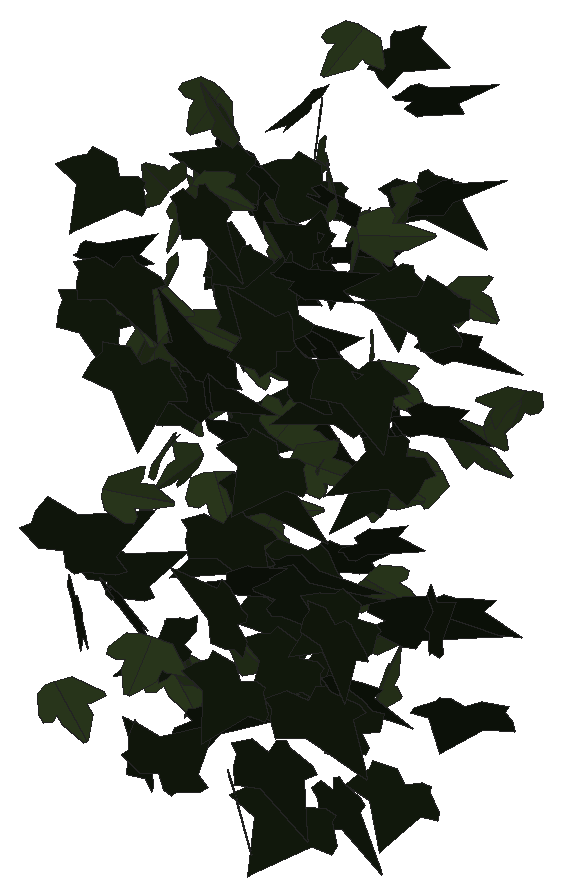
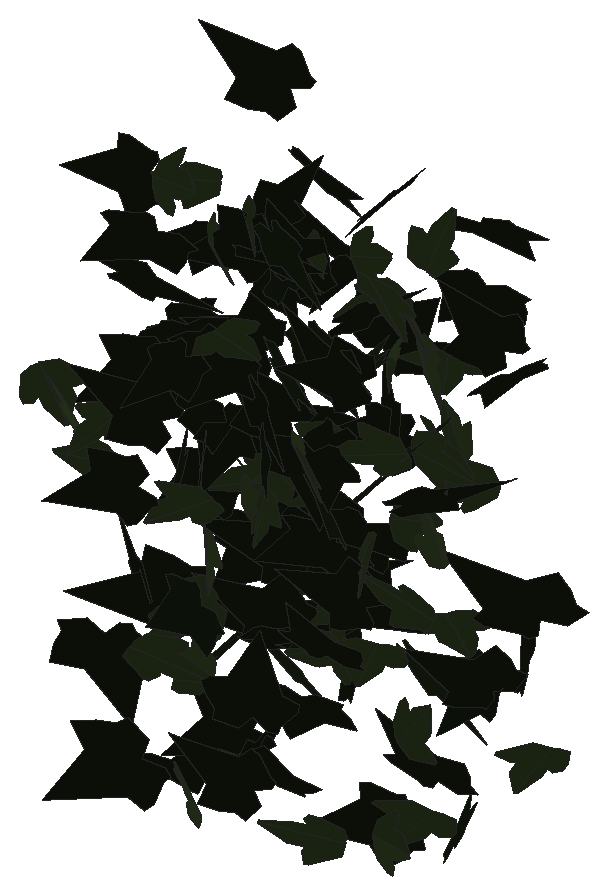
# SketchUp Ruby script. Lengths in inches.
U = 1.inch
M = Sketchup.active_model
def pt(a) = Geom::Point3d.new(a.map { |v| v * U })
def face(e, loops, mat)
  f = e.add_face(loops[0].map { |a| pt(a) })
  loops[1..].each { |l| e.add_face(l.map { |a| pt(a) }).erase! }
  f.material = f.back_material = mat if mat
  f
end
# faces: each face lists its corners as indices into pts; further lists are holes
def faces(e, pts, list, mat = nil) = list.each { |f| face(e, (f[0].is_a?(Array) ? f : [f]).map { |l| l.map { |i| pts[i] } }, mat) }
# xy, xz, yz: faces in a plane at the given z, y or x. An outline is a flat list of corners, or four numbers for a rectangle; further outlines are holes
def ring(l) = l.size == 4 ? [[l[0], l[1]], [l[2], l[1]], [l[2], l[3]], [l[0], l[3]]] : l.each_slice(2).to_a
def flat(e, list, mat, &to3) = list.each { |f| face(e, (f[0].is_a?(Array) ? f : [f]).map { |l| ring(l).map { |u, v| to3.(u, v) } }, mat) }
def xy(e, z, list, mat = nil) = flat(e, list, mat) { |x, y| [x, y, z] }
def xz(e, y, list, mat = nil) = flat(e, list, mat) { |x, z| [x, y, z] }
def yz(e, x, list, mat = nil) = flat(e, list, mat) { |y, z| [x, y, z] }
def lines(e, pts, list) = list.each { |a, b| e.add_line(pt(pts[a]), pt(pts[b])) }
# prism: a flat outline (further loops are holes) pulled along v
def prism(e, loops, v, mat = nil)
  f = face(e, loops, mat); d = Geom::Vector3d.new(v.map { |x| x * U })
  f.pushpull(f.normal.samedirection?(d) ? d.length : -d.length)
end
def box(e, o, s, mat = nil) = prism(e, [[o, [o[0] + s[0], o[1], o[2]], [o[0] + s[0], o[1] + s[1], o[2]], [o[0], o[1] + s[1], o[2]]]], [0, 0, s[2]], mat)
def at(x, y, z, deg = 0) = Geom::Transformation.translation(pt([x, y, z])) * Geom::Transformation.rotation(ORIGIN, Z_AXIS, deg.degrees)
def axes(o, x, y, z) = Geom::Transformation.new([*x, 0, *y, 0, *z, 0, *pt(o).to_a, 1])
def part(name) = M.definitions.add(name)
# library, detail: a bought-in or finely detailed component or shape, given as its bounding box
def library(name, o, s) = part(name).tap { |d| box(d.entities, o, s) }
def detail(e, o, s) = box(e.add_group.entities, o, s)
def put(e, d, t, mat = nil) = e.add_instance(d, t).tap { |i| i.material = mat if mat }
def group(e, t, mat = nil) = e.add_group.tap { |g| g.transformation = t; g.material = mat if mat }.entities
root = M.entities
M.materials.add("1026 AP 7946 SUNNY SIDE UP").color = [254, 231, 186]
M.materials.add("efeu1").color = [18, 25, 13]
M.materials.add("efeu2").color = [43, 57, 29]
c1 = part("ivyleaf_10")
p = [[0,0.5,-0.03],[-0.0625,2.02,-0.43],[-0.19,2.01,-0.46],[-0.54,1.05,-0.29],[-0.52,0.625,-0.18],[-0.83,0.76,-0.28],
  [-1.16,0.64,-0.33],[-1.15,0.33,-0.24],[-0.77,-0.39,0.02],[-0.3,-0.51,0.16],[0.04,-0.48,0.23],[-0.02,2.01,-0.4375],
  [-0.06,2.01,-0.43],[0.04,-0.49,0.23],[0.67,-0.49,0.14],[1.38,0.36,-0.2],[1.375,0.51,-0.24],[0.81,0.65,-0.19],
  [0.62,0.59,-0.15],[0.6,1.09,-0.28],[0.5,1.23,-0.31]]
faces(c1.entities,p,[[0,1,2,3,4,5,6,7,8,9,10],[11,12,0,13,14,15,16,17,18,19,20]],"efeu2")
c2 = part("ivyleaf_9")
p = [[1.54,2.16,1.25],[1.36,2.04,1.19],[-0.21,0.99,0.68],[-0.71,1.11,0.82],[-0.85,0.86,0.67],[-0.8,0.17,0.21],
  [-0.9,-0.01,0.1],[-0.67,-0.16,-0.02],[-0.08,-0.08,-0.05],[-0.03,-0.6,-0.4],[0.65,-0.88,-0.66],[0.83,-0.6,-0.49],
  [1.29,-0.42,-0.43],[1.8125,-0.07,-0.26],[1.21,0.44,0.15]]
faces(c2.entities,p,[[0,1,2,3,4,5,6,7,8,9,10,11,12,13,14]],"efeu1")
put(root,c1,axes([150.24,214.86,288],[0.00034,-0.24458,-0.28841],[0.01461,0.27848,-0.25025],[0.58271,-0.00684,0.00644]),"1026 AP 7946 SUNNY SIDE UP")
put(root,c1,axes([150.29,212.04,290.43],[0.54174,-0.1658,-0.09106],[-0.13351,0.0251,-0.39349],[0.26277,0.35457,-0.01218]),"1026 AP 7946 SUNNY SIDE UP")
put(root,c2,axes([149.95,209.48,288.4],[0.45459,0.23395,-0.02201],[-0.00198,0.03751,0.38211],[0.36958,-0.28756,0.02911]),"1026 AP 7946 SUNNY SIDE UP")
put(root,c2,axes([150.08,209.08,287.71],[0.00627,-0.39476,-0.09926],[0.00472,0.09414,-0.40613],[0.6381,0.00318,0.00398]),"1026 AP 7946 SUNNY SIDE UP")
put(root,c1,axes([150.71,210.34,286.64],[-0.04708,-0.01723,-0.40837],[-0.50973,0.23012,0.01627],[0.35949,0.32404,-0.03041]),"1026 AP 7946 SUNNY SIDE UP")
put(root,c1,axes([149.87,213.81,281.72],[0.10364,-0.0263,-0.38331],[0.56164,0.11278,0.05766],[0.16815,-0.36049,0.04368]),"1026 AP 7946 SUNNY SIDE UP")
put(root,c1,axes([150.11,208.24,280.67],[0.29267,0.32134,0.13775],[0.1212,0.10769,-0.38173],[-0.53256,0.2011,-0.01118]),"1026 AP 7946 SUNNY SIDE UP")
put(root,c1,axes([149.9,211.58,284.72],[0.1979,-0.0697,-0.35915],[0.53898,-0.07279,0.14221],[-0.14605,-0.36305,0.03816]),"1026 AP 7946 SUNNY SIDE UP")
put(root,c2,axes([150.51,209.19,290.25],[-0.54504,-0.1927,-0.01598],[0.05045,-0.0282,-0.40663],[0.29963,-0.34578,0.0394]),"1026 AP 7946 SUNNY SIDE UP")
put(root,c2,axes([149.99,208.55,283.28],[-0.17111,0.04006,0.48252],[0.73686,-0.02559,0.11433],[0.05358,0.47995,-0.03134]),"1026 AP 7946 SUNNY SIDE UP")
put(root,c1,axes([150.58,211.34,288.83],[-0.03018,0.18451,-0.32659],[-0.14274,0.30626,0.19046],[0.56028,0.08796,0.03093]),"1026 AP 7946 SUNNY SIDE UP")
put(root,c2,axes([150.23,214.96,288.8125],[-0.09888,-0.02115,-0.37658],[0.4884,-0.19924,-0.04435],[-0.3045,-0.31271,0.05115]),"1026 AP 7946 SUNNY SIDE UP")
put(root,c2,axes([150.18,209.46,282.35],[-0.04219,0.03422,0.41272],[0.61861,0.08419,0.02024],[-0.12905,0.3924,-0.03791]),"1026 AP 7946 SUNNY SIDE UP")
put(root,c2,axes([150.21,208.48,282.41],[0.17647,-0.13219,-0.39528],[0.52913,-0.19083,0.16834],[-0.35468,-0.35046,0.05448]),"1026 AP 7946 SUNNY SIDE UP")
put(root,c2,axes([150.96,210.46,285.75],[-0.2897,-0.40546,-0.16511],[-0.13991,-0.13281,0.45733],[-0.66977,0.20312,-0.02412]),"1026 AP 7946 SUNNY SIDE UP")
put(root,c1,axes([150.59,209.72,286.52],[0.02737,-0.37422,-0.00824],[0.00724,-0.00567,0.38588],[-0.58846,-0.01748,0.00436]),"1026 AP 7946 SUNNY SIDE UP")
put(root,c2,axes([150.47,209.22,282.26],[0.55635,-0.13712,-0.12245],[-0.19009,0.01383,-0.38967],[0.21172,0.37275,-0.02811]),"1026 AP 7946 SUNNY SIDE UP")
put(root,c2,axes([150.28,212.57,289.06],[0.42377,-0.12014,0.22844],[0.30943,-0.10439,-0.30434],[0.24953,0.33349,-0.01057]),"1026 AP 7946 SUNNY SIDE UP")
put(root,c1,axes([150.6,210.05,286.77],[0.51821,-0.16541,0.14391],[0.17496,-0.09084,-0.37922],[0.29316,0.34661,-0.02808]),"1026 AP 7946 SUNNY SIDE UP")
put(root,c1,axes([150.82,210.6,289.13],[0.3492,-0.30517,0.07536],[0.04115,-0.07341,-0.38861],[0.49237,0.22257,-0.02097]),"1026 AP 7946 SUNNY SIDE UP")
put(root,c1,axes([151.16,211.37,290.43],[-0.20983,0.13808,-0.3234],[-0.33943,0.22901,0.19915],[0.42048,0.25377,-0.00062]),"1026 AP 7946 SUNNY SIDE UP")
put(root,c2,axes([150.6,210.57,287],[0.10705,-0.39481,0.05601],[0.00608,-0.05678,-0.41303],[0.62712,0.06795,-0.00556]),"1026 AP 7946 SUNNY SIDE UP")
put(root,c1,axes([150.93,211.48,285.47],[-0.25567,0.31194,0.16328],[-0.1495,0.12678,-0.36084],[-0.52816,-0.18689,0.0231]),"1026 AP 7946 SUNNY SIDE UP")
put(root,c1,axes([150.9375,209.99,289.87],[-0.14488,-0.27499,-0.27658],[-0.16628,-0.24561,0.29686],[-0.57918,0.1393,-0.01604]),"1026 AP 7946 SUNNY SIDE UP")
put(root,c1,axes([150.96,210.08,288.21],[0.17104,-0.3806,-0.06422],[-0.05174,0.05313,-0.40711],[0.60368,0.11239,-0.01669]),"1026 AP 7946 SUNNY SIDE UP")
put(root,c2,axes([151.11,212.31,286.45],[0.00976,0.18092,0.35437],[-0.05752,0.34175,-0.18304],[-0.60699,-0.02948,0.02305]),"1026 AP 7946 SUNNY SIDE UP")
put(root,c1,axes([150.63,210.48,280.4],[0.45779,0.21342,0.1689],[0.24019,0.06566,-0.36984],[-0.347,0.32701,-0.03317]),"1026 AP 7946 SUNNY SIDE UP")
put(root,c2,axes([151.17,211.74,289.44],[-0.06207,-0.33555,-0.20129],[0.00563,-0.19479,0.34613],[-0.60902,0.0324,0.02372]),"1026 AP 7946 SUNNY SIDE UP")
put(root,c1,axes([151.09,214.87,290.61],[0.32558,0.21594,-0.25711],[-0.23061,-0.20533,-0.30807],[-0.4665,0.25221,-0.02714]),"1026 AP 7946 SUNNY SIDE UP")
put(root,c1,axes([150.86,209.91,284.68],[0.09622,-0.35154,-0.13633],[0.10498,-0.11973,0.36429],[-0.58011,-0.07998,0.04331]),"1026 AP 7946 SUNNY SIDE UP")
put(root,c1,axes([150.99,211.06,280.11],[0.1059,-0.23251,0.30563],[0.11783,-0.28846,-0.251],[0.58252,0.10062,-0.00479]),"1026 AP 7946 SUNNY SIDE UP")
put(root,c2,axes([150.93,209.38,279.36],[-0.0516,-0.14945,0.37337],[-0.07555,-0.36028,-0.15927],[0.61303,-0.05698,0.0118]),"1026 AP 7946 SUNNY SIDE UP")
put(root,c1,axes([150.91,209.57,287.91],[0.48108,0.21701,0.02587],[0.05927,-0.01202,-0.38513],[-0.33813,0.30665,-0.03071]),"1026 AP 7946 SUNNY SIDE UP")
put(root,c2,axes([150.96,212.49,284.02],[-0.41082,0.1446,0.22534],[0.32976,-0.06821,0.30525],[0.2457,0.33331,-0.03289]),"1026 AP 7946 SUNNY SIDE UP")
put(root,c2,axes([151.13,215.4,286.07],[-0.18298,0.24576,-0.30283],[-0.16397,0.27681,0.28124],[0.58148,0.15539,-0.01599]),"1026 AP 7946 SUNNY SIDE UP")
put(root,c1,axes([150.94,211.35,283.58],[0.45385,0.25447,0.08235],[0.12239,0.03009,-0.39516],[-0.40045,0.2976,-0.02744]),"1026 AP 7946 SUNNY SIDE UP")
put(root,c2,axes([150.875,208.71,288.81],[-0.22082,-0.19079,-0.33081],[0.34068,0.23642,-0.24176],[0.47662,-0.25738,0.01955]),"1026 AP 7946 SUNNY SIDE UP")
put(root,c2,axes([150.77,212.36,288.68],[-0.05022,0.0705,0.4441],[0.37785,-0.35763,0.07658],[0.57282,0.24209,-0.01158]),"1026 AP 7946 SUNNY SIDE UP")
put(root,c1,axes([151.26,212.72,287.52],[0.36743,-0.32066,0.03108],[0.00066,-0.03922,-0.40831],[0.5067,0.23257,-0.02201]),"1026 AP 7946 SUNNY SIDE UP")
put(root,c1,axes([151.07,210.81,289.52],[-0.19708,-0.15266,-0.31964],[0.3999,0.18157,-0.19736],[0.3666,-0.28013,0.04345]),"1026 AP 7946 SUNNY SIDE UP")
put(root,c2,axes([151.29,211.375,288.16],[-0.2015,-0.26233,0.30728],[-0.06883,-0.30371,-0.29487],[0.62256,-0.11848,0.06685]),"1026 AP 7946 SUNNY SIDE UP")
put(root,c2,axes([151.48,212.14,287.16],[0.30508,0.27098,-0.16444],[-0.14239,-0.13335,-0.3441],[-0.47485,0.21408,-0.00246]),"1026 AP 7946 SUNNY SIDE UP")
put(root,c1,axes([151.01,210.85,286.8],[0.13389,0.09764,0.36147],[0.43736,0.2143,-0.12993],[-0.3684,0.28991,-0.02289]),"1026 AP 7946 SUNNY SIDE UP")
put(root,c1,axes([151.7,209.58,281.05],[-0.44068,0.20269,-0.19714],[-0.21039,0.14208,0.35561],[0.38593,0.3089,-0.03125]),"1026 AP 7946 SUNNY SIDE UP")
put(root,c2,axes([151.46,211.36,288.15],[-0.25654,-0.18391,0.34807],[-0.09845,-0.35048,-0.22904],[0.59826,-0.13654,0.11156]),"1026 AP 7946 SUNNY SIDE UP")
put(root,c2,axes([151.44,215.4,290.29],[0.03416,-0.00028,-0.40229],[-0.16016,0.37756,-0.0039],[0.59276,0.10203,0.02213]),"1026 AP 7946 SUNNY SIDE UP")
put(root,c2,axes([151.05,211.49,284.39],[0.29873,-0.08382,0.32586],[0.43791,-0.15166,-0.21429],[0.27152,0.33682,-0.0129]),"1026 AP 7946 SUNNY SIDE UP")
put(root,c1,axes([151.59,209.82,284.95],[0.01963,-0.11739,0.37353],[0.04799,-0.36198,-0.1237],[0.59834,0.03288,-0.00233]),"1026 AP 7946 SUNNY SIDE UP")
put(root,c1,axes([151.35,208.21,284.95],[0.05812,0.09763,0.39619],[0.18914,0.36472,-0.10532],[-0.59365,0.12576,0.00523]),"1026 AP 7946 SUNNY SIDE UP")
put(root,c2,axes([151.54,213.5625,283.24],[0.5902,-0.11463,0.14851],[-0.18939,0.09673,0.40106],[-0.22015,-0.39052,0.05313]),"1026 AP 7946 SUNNY SIDE UP")
put(root,c2,axes([152.08,208.95,281.98],[-0.52423,0.31035,-0.04182],[0.01308,-0.05307,-0.46832],[-0.49235,-0.33186,0.03209]),"1026 AP 7946 SUNNY SIDE UP")
put(root,c2,axes([151.52,210.0625,279.86],[0.06074,0.21571,-0.37049],[0.04708,0.36004,0.22714],[0.65938,-0.04558,0.01791]),"1026 AP 7946 SUNNY SIDE UP")
put(root,c2,axes([151.68,208.4,287.38],[-0.27135,-0.41978,-0.06538],[0.05889,0.05061,-0.46701],[0.66442,-0.17592,0.01469]),"1026 AP 7946 SUNNY SIDE UP")
put(root,c2,axes([151.88,211.18,286.92],[0.0224,-0.07632,-0.39385],[-0.27179,0.34119,-0.0749],[0.54872,0.17211,-0.02102]),"1026 AP 7946 SUNNY SIDE UP")
put(root,c2,axes([152.14,212.28,290.83],[-0.28555,0.31398,-0.0678],[0.03102,-0.0666,-0.37369],[-0.50406,-0.18197,0.01541]),"1026 AP 7946 SUNNY SIDE UP")
put(root,c2,axes([151.82,209.85,286.46],[-0.10023,0.0846,0.38387],[0.02068,-0.37658,0.08832],[0.59972,0.02713,0.06111]),"1026 AP 7946 SUNNY SIDE UP")
put(root,c2,axes([151.65,209.73,286.4],[0.14159,0.06583,-0.37095],[0.26469,0.32225,0.10584],[0.51175,-0.1849,0.04789]),"1026 AP 7946 SUNNY SIDE UP")
put(root,c1,axes([152.05,208.09,282.29],[0.48956,0.21843,-0.12527],[-0.1272,-0.09782,-0.39099],[-0.37296,0.32008,-0.03109]),"1026 AP 7946 SUNNY SIDE UP")
put(root,c2,axes([151.72,215.67,289.27],[0.37197,0.28969,-0.14248],[0.10344,0.12649,0.38502],[0.49519,-0.24403,0.0266]),"1026 AP 7946 SUNNY SIDE UP")
put(root,c2,axes([152.38,211.11,288.43],[-0.26821,0.33573,-0.12566],[0.06427,-0.11806,-0.38828],[-0.55902,-0.17466,0.01565]),"1026 AP 7946 SUNNY SIDE UP")
put(root,c2,axes([152.44,210.15,283.42],[-0.03046,0.0007,-0.38449],[-0.09435,-0.36887,0.00034],[-0.57923,0.06005,0.02016]),"1026 AP 7946 SUNNY SIDE UP")
put(root,c2,axes([151.98,208.53,279.75],[-0.32798,0.16399,0.33139],[0.44559,-0.15413,0.27013],[0.34971,0.35019,-0.03339]),"1026 AP 7946 SUNNY SIDE UP")
put(root,c2,axes([151.85,213.24,281.67],[0.40431,0.23872,-0.12941],[0.10877,0.11131,0.36056],[0.41101,-0.26429,0.03188]),"1026 AP 7946 SUNNY SIDE UP")
put(root,c2,axes([152.58,212.29,287.9375],[0.07429,-0.03393,-0.39955],[-0.60489,0.05473,-0.05292],[0.09215,0.38666,-0.02525]),"1026 AP 7946 SUNNY SIDE UP")
put(root,c2,axes([152.53,209.07,287.35],[0.30089,-0.16706,0.39356],[-0.39102,0.29297,0.26137],[-0.52796,-0.31218,0.03072]),"1026 AP 7946 SUNNY SIDE UP")
put(root,c1,axes([152.22,210.89,286.68],[0.05329,0.22926,0.30786],[0.11035,0.28962,-0.23644],[-0.58022,0.07613,-0.01669]),"1026 AP 7946 SUNNY SIDE UP")
put(root,c2,axes([152.16,209.3125,290.29],[0.24225,-0.38218,-0.16429],[-0.08259,0.14841,-0.42359],[0.64459,0.16265,0.00747]),"1026 AP 7946 SUNNY SIDE UP")
put(root,c1,axes([152.35,210.53,283.46],[-0.0079,-0.18662,-0.35872],[0.21564,0.32466,-0.17995],[0.58101,-0.12303,0.06191]),"1026 AP 7946 SUNNY SIDE UP")
put(root,c1,axes([152.625,213.29,285.76],[0.07758,-0.26003,-0.30807],[-0.09268,0.29168,-0.27094],[0.61442,0.07683,-0.00197]),"1026 AP 7946 SUNNY SIDE UP")
put(root,c2,axes([152.64,211.61,288.17],[-0.43506,0.13387,-0.26074],[0.32748,-0.14895,-0.31564],[-0.31049,-0.34469,0.03243]),"1026 AP 7946 SUNNY SIDE UP")
put(root,c2,axes([152.9,211.59,289.9375],[-0.5775,-0.13971,-0.0161],[0.04372,-0.03157,-0.40296],[0.21655,-0.36621,0.03841]),"1026 AP 7946 SUNNY SIDE UP")
put(root,c2,axes([152.64,211.01,281.99],[-0.38639,-0.22147,-0.2368],[0.28823,0.13764,-0.33955],[0.40916,-0.3061,0.01557]),"1026 AP 7946 SUNNY SIDE UP")
put(root,c2,axes([152.64,209.79,289.1],[0.06317,-0.30765,-0.25524],[-0.07814,0.24136,-0.31789],[0.61446,0.06232,-0.01419]),"1026 AP 7946 SUNNY SIDE UP")
put(root,c2,axes([152.4375,210.48,284.5625],[-0.04959,-0.0723,-0.40202],[0.42664,0.2812,-0.0747],[0.45455,-0.27182,0.02625]),"1026 AP 7946 SUNNY SIDE UP")
put(root,c1,axes([152.71,210.95,285.46],[0.57281,-0.01251,-0.15448],[0.2347,0.07846,0.36743],[0.02914,-0.38602,0.07733]),"1026 AP 7946 SUNNY SIDE UP")
put(root,c2,axes([152.7,209.35,284.28],[-0.19148,-0.20828,-0.34394],[0.31857,0.26497,-0.24575],[0.52859,-0.23514,0.02352]),"1026 AP 7946 SUNNY SIDE UP")
put(root,c2,axes([153.36,210.96,282.76],[-0.39721,-0.29197,-0.08004],[-0.10897,-0.04036,0.39664],[-0.46172,0.2607,-0.02475]),"1026 AP 7946 SUNNY SIDE UP")
put(root,c1,axes([152.61,210.67,289.44],[-0.08577,0.02848,0.37617],[0.54974,-0.10538,0.06168],[0.17071,0.35367,-0.00965]),"1026 AP 7946 SUNNY SIDE UP")
put(root,c1,axes([153.46,213.7,283.69],[0.27,-0.00715,-0.37068],[-0.55812,-0.06893,-0.17351],[-0.09306,0.39265,-0.03484]),"1026 AP 7946 SUNNY SIDE UP")
put(root,c2,axes([152.67,211.33,287.04],[0.5461,0.06124,-0.17257],[0.23772,0.09489,0.35844],[0.14977,-0.37389,0.06031]),"1026 AP 7946 SUNNY SIDE UP")
put(root,c2,axes([152.78,210.67,289.17],[-0.07401,0.02993,0.45518],[0.33888,-0.38642,0.04838],[0.60802,0.21902,0.02844]),"1026 AP 7946 SUNNY SIDE UP")
put(root,c2,axes([153,212.29,288.4],[0.44685,0.25861,0.08693],[0.11505,0.04266,-0.39519],[-0.41124,0.29294,-0.0161]),"1026 AP 7946 SUNNY SIDE UP")
put(root,c2,axes([153.49,210.81,280.27],[-0.60451,0.07231,0.09048],[0.1449,0.01889,0.40152],[0.10405,0.39381,-0.03349]),"1026 AP 7946 SUNNY SIDE UP")
put(root,c1,axes([153.59,211.09,290.1],[0.0152,-0.06857,-0.40183],[-0.20301,0.36789,-0.06784],[0.58806,0.12877,-0.01303]),"1026 AP 7946 SUNNY SIDE UP")
put(root,c2,axes([153.28,208.74,283.75],[0.39199,0.30613,0.1433],[0.15752,0.09541,-0.4058],[-0.50353,0.26817,-0.0154]),"1026 AP 7946 SUNNY SIDE UP")
put(root,c2,axes([153.21,210.62,288.875],[-0.00822,-0.17207,0.33736],[0.12837,-0.32095,-0.17376],[0.56873,0.06996,0.04409]),"1026 AP 7946 SUNNY SIDE UP")
put(root,c1,axes([153.2,209.4375,282.01],[-0.36282,0.02081,-0.29544],[0.43799,-0.07566,-0.23688],[-0.11292,-0.36032,0.03047]),"1026 AP 7946 SUNNY SIDE UP")
put(root,c2,axes([153.66,211.14,280.36],[-0.07359,0.07573,0.44929],[-0.36458,-0.37727,0.03969],[0.59211,-0.22289,0.08028]),"1026 AP 7946 SUNNY SIDE UP")
put(root,c1,axes([153.5,211.15,285.04],[-0.01211,-0.11245,-0.38931],[0.01544,-0.37727,0.11344],[-0.61881,-0.00721,0.01045]),"1026 AP 7946 SUNNY SIDE UP")
put(root,c2,axes([153.76,209.39,285.93],[-0.53925,-0.18869,-0.02745],[0.06026,-0.0168,-0.4019],[0.29328,-0.34349,0.03211]),"1026 AP 7946 SUNNY SIDE UP")
put(root,c2,axes([153.94,211.12,286.4],[-0.05498,0.00363,-0.40536],[-0.12291,-0.38724,0.00121],[-0.60643,0.07815,0.0365]),"1026 AP 7946 SUNNY SIDE UP")
put(root,c2,axes([153.26,211.31,289.85],[0.54075,-0.06966,0.13793],[0.19788,-0.05334,-0.36084],[0.13201,0.36531,-0.02412]),"1026 AP 7946 SUNNY SIDE UP")
put(root,c1,axes([153.35,212.625,285.89],[0.24219,0.19607,0.29536],[0.32655,0.1979,-0.25419],[-0.43598,0.25714,-0.02632]),"1026 AP 7946 SUNNY SIDE UP")
put(root,c2,axes([153.73,209.02,288.6],[-0.6018,0.17905,0.18939],[0.2898,-0.03532,0.4329],[0.27914,0.42268,-0.04112]),"1026 AP 7946 SUNNY SIDE UP")
put(root,c2,axes([153.26,210.62,282.91],[0.18576,-0.08171,0.37857],[0.55336,-0.11415,-0.14319],[0.21219,0.3692,0.04199]),"1026 AP 7946 SUNNY SIDE UP")
put(root,c2,axes([153.92,210.11,289.62],[0.06264,0.06965,0.39797],[-0.44777,-0.26154,0.07738],[0.42392,-0.28654,0.02293]),"1026 AP 7946 SUNNY SIDE UP")
put(root,c1,axes([153.66,212.21,284.03],[-0.06909,-0.1516,-0.35305],[0.33054,0.27465,-0.15171],[0.4863,-0.20822,0.05296]),"1026 AP 7946 SUNNY SIDE UP")
put(root,c1,axes([153.77,212.25,280.27],[0.38203,-0.30915,0.04578],[-0.01455,0.05137,0.40459],[-0.49129,-0.24192,0.02362]),"1026 AP 7946 SUNNY SIDE UP")
put(root,c2,axes([154.07,207.88,283.59],[-0.02274,-0.42804,0.02531],[0.00056,0.027,0.44137],[-0.67439,0.01445,-0.00048]),"1026 AP 7946 SUNNY SIDE UP")
put(root,c2,axes([154.27,209.48,281.5],[-0.4811,0.26375,0.03233],[-0.06883,-0.00516,-0.41484],[-0.41166,-0.30737,0.03158]),"1026 AP 7946 SUNNY SIDE UP")
put(root,c1,axes([153.59,210.43,285.3125],[0.10247,0.12198,0.39182],[0.34158,0.31173,-0.13978],[-0.52581,0.22628,-0.01444]),"1026 AP 7946 SUNNY SIDE UP")
put(root,c2,axes([154.06,207.98,282.4],[-0.33926,-0.33419,0.09959],[-0.05488,-0.09463,-0.40976],[0.54511,-0.21752,0.02073]),"1026 AP 7946 SUNNY SIDE UP")
put(root,c2,axes([154.05,211.08,286.35],[0.52831,0.0195,-0.18851],[-0.28227,-0.05002,-0.34516],[-0.06438,0.37935,-0.03356]),"1026 AP 7946 SUNNY SIDE UP")
put(root,c1,axes([153.96,211.43,289.625],[0.30819,-0.23008,0.26998],[0.22226,-0.22403,-0.3113],[0.50298,0.23998,-0.02786]),"1026 AP 7946 SUNNY SIDE UP")
put(root,c2,axes([153.82,210.81,280.96],[0.55156,0.08609,0.15429],[0.23984,0.00244,-0.37066],[-0.1261,0.38121,-0.03013]),"1026 AP 7946 SUNNY SIDE UP")
put(root,c2,axes([154.1,211.96,288.43],[-0.21924,-0.35513,-0.13609],[0.09522,0.11589,-0.39212],[0.58701,-0.15144,0.01278]),"1026 AP 7946 SUNNY SIDE UP")
put(root,c2,axes([154.4,211.17,286.07],[0.19909,-0.11256,-0.35621],[-0.47818,0.16673,-0.16998],[0.31173,0.32764,-0.03324]),"1026 AP 7946 SUNNY SIDE UP")
put(root,c2,axes([153.89,213.52,286.36],[0.48286,0.08415,0.21427],[0.32855,0.01898,-0.32636],[-0.12663,0.37014,-0.02969]),"1026 AP 7946 SUNNY SIDE UP")
put(root,c2,axes([153.8,210.52,287.5],[0.39637,-0.21193,0.3069],[0.32263,-0.21925,-0.33946],[0.47766,0.32395,-0.02539]),"1026 AP 7946 SUNNY SIDE UP")
put(root,c2,axes([154.44,209.07,282.49],[-0.36831,-0.29057,0.1667],[-0.11554,-0.14987,-0.38379],[0.51134,-0.24316,0.03335]),"1026 AP 7946 SUNNY SIDE UP")
put(root,c2,axes([154.04,213.26,281.42],[0.53574,0.23123,0.22734],[0.31065,0.09876,-0.42279],[-0.39327,0.393,-0.02427]),"1026 AP 7946 SUNNY SIDE UP")
put(root,c2,axes([153.85,209.37,283.3125],[0.21263,0.02516,0.43615],[0.66665,-0.00939,-0.13904],[0.00205,0.4442,-0.02504]),"1026 AP 7946 SUNNY SIDE UP")
put(root,c2,axes([154.87,207.92,289.08],[-0.51791,0.04324,-0.25185],[-0.37946,0.04128,0.34238],[0.09322,0.40825,-0.0055]),"1026 AP 7946 SUNNY SIDE UP")
put(root,c1,axes([154.34,213.52,287.44],[0.11365,0.24729,0.29091],[0.0898,0.27553,-0.26334],[-0.58166,0.09086,0.01618]),"1026 AP 7946 SUNNY SIDE UP")
put(root,c2,axes([154.37,211.96,285.35],[-0.01334,-0.08676,0.45351],[-0.09739,-0.43635,-0.09227],[0.69953,-0.0624,-0.0042]),"1026 AP 7946 SUNNY SIDE UP")
put(root,c1,axes([154.47,211.19,281.9],[0.07556,-0.28649,0.25506],[0.06286,0.25362,0.2939],[-0.59374,-0.00961,0.06357]),"1026 AP 7946 SUNNY SIDE UP")
put(root,c2,axes([154.22,209.23,287.68],[-0.01429,0.05477,0.43067],[0.501,-0.27249,0.04235],[0.43345,0.31676,-0.03475]),"1026 AP 7946 SUNNY SIDE UP")
put(root,c1,axes([154.4375,211.18,283.01],[-0.20433,-0.20735,-0.30605],[0.39213,0.17608,-0.2389],[0.41112,-0.271,0.07575]),"1026 AP 7946 SUNNY SIDE UP")
put(root,c2,axes([154.33,207.58,280.51],[0.19559,-0.12682,-0.43772],[0.61416,-0.17599,0.17118],[-0.32774,-0.40549,0.05955]),"1026 AP 7946 SUNNY SIDE UP")
put(root,c2,axes([154.48,212.29,290.08],[-0.0761,-0.11262,-0.39029],[0.33131,0.31481,-0.12251],[0.52465,-0.21513,0.02075]),"1026 AP 7946 SUNNY SIDE UP")
put(root,c1,axes([154.99,211.41,290.42],[0.04049,-0.21014,0.35325],[0.12021,-0.33599,-0.21925],[0.62247,0.07856,0.01936]),"1026 AP 7946 SUNNY SIDE UP")
put(root,c2,axes([155.25,210.21,285.62],[-0.5347,0.09847,-0.14508],[0.19373,-0.07972,-0.36293],[-0.1894,-0.35954,0.03837]),"1026 AP 7946 SUNNY SIDE UP")
put(root,c2,axes([155.4375,209.36,283.47],[-0.53074,-0.13602,0.09247],[-0.10692,-0.072,-0.37303],[0.23361,-0.34197,0.03935]),"1026 AP 7946 SUNNY SIDE UP")
put(root,c1,axes([154.87,210.58,290.08],[0.09203,-0.05221,-0.3785],[0.51133,0.18582,0.02727],[0.28018,-0.32198,0.07455]),"1026 AP 7946 SUNNY SIDE UP")
put(root,c2,axes([155.74,209.08,281.5625],[-0.24914,0.04765,0.34667],[-0.53251,0.0055,-0.16517],[-0.03982,-0.37166,0.03979]),"1026 AP 7946 SUNNY SIDE UP")
put(root,c2,axes([155.1,209.99,284.54],[0.33849,0.23351,0.21885],[0.25534,0.13673,-0.32559],[-0.42405,0.26873,-0.02135]),"1026 AP 7946 SUNNY SIDE UP")
put(root,c2,axes([155.89,211.3,288.43],[-0.41131,0.0993,0.29499],[-0.4407,0.06271,-0.28637],[-0.17912,-0.38231,0.0272]),"1026 AP 7946 SUNNY SIDE UP")
put(root,c2,axes([155.46,210.625,279.74],[-0.43125,-0.26247,-0.06484],[0.099,0.02287,-0.38998],[0.41215,-0.28013,0.02583]),"1026 AP 7946 SUNNY SIDE UP")
put(root,c2,axes([155.28,211.48,290.49],[0.06559,0.2895,-0.27569],[0.01609,0.26987,0.30213],[0.62145,-0.03754,0.02128]),"1026 AP 7946 SUNNY SIDE UP")
put(root,c2,axes([155.09,210.75,282.72],[0.42032,0.08369,0.39075],[0.58964,0.0622,-0.28639],[-0.15639,0.45945,-0.02958]),"1026 AP 7946 SUNNY SIDE UP")
put(root,c2,axes([155.44,208.19,282.39],[-0.15675,-0.21201,-0.37827],[0.29633,0.31435,-0.23865],[0.59538,-0.21228,0.01919]),"1026 AP 7946 SUNNY SIDE UP")
put(root,c2,axes([155.875,207.39,280.88],[-0.59975,-0.26562,0.00874],[0.02469,-0.03997,-0.47713],[0.41723,-0.37945,0.0408]),"1026 AP 7946 SUNNY SIDE UP")
put(root,c2,axes([155.33,208.02,290.46],[0.51108,0.20771,-0.1505],[0.16584,0.10753,0.39667],[0.3644,-0.34025,0.03056]),"1026 AP 7946 SUNNY SIDE UP")
put(root,c1,axes([155.46,212.24,285.67],[-0.21169,0.03522,-0.3661],[0.50718,-0.1515,-0.14216],[-0.24172,-0.34872,0.02234]),"1026 AP 7946 SUNNY SIDE UP")
put(root,c2,axes([155.67,209.19,288.31],[-0.2198,-0.32549,-0.23639],[0.16092,0.20363,-0.36355],[0.60344,-0.17286,0.01084]),"1026 AP 7946 SUNNY SIDE UP")
put(root,c2,axes([155.54,210.875,286.7],[0.49537,0.1758,0.17877],[0.26808,0.04654,-0.3693],[-0.27954,0.35616,-0.03736]),"1026 AP 7946 SUNNY SIDE UP")
put(root,c2,axes([155.71,208.51,283.79],[0.02546,-0.41307,0.10351],[0.00359,-0.10281,-0.42647],[0.66933,0.01626,-0.00165]),"1026 AP 7946 SUNNY SIDE UP")
put(root,c2,axes([156.24,209.66,286.71],[-0.02417,-0.06191,-0.449],[0.04913,-0.43481,0.06],[-0.68991,-0.0288,0.02]),"1026 AP 7946 SUNNY SIDE UP")
put(root,c2,axes([155.89,210.83,282.77],[-0.06278,0.19219,0.35899],[0.07018,-0.34475,0.19975],[0.62029,0.05845,0.01373]),"1026 AP 7946 SUNNY SIDE UP")
put(root,c2,axes([155.94,208.23,280.82],[0.30465,-0.36972,-0.12318],[-0.07733,0.10684,-0.42935],[0.60506,0.19981,0.00715]),"1026 AP 7946 SUNNY SIDE UP")
put(root,c2,axes([155.99,206.43,282.36],[-0.30149,-0.11565,-0.39993],[0.57391,0.13529,-0.22683],[0.27396,-0.41068,0.03505]),"1026 AP 7946 SUNNY SIDE UP")
put(root,c1,axes([156.11,212.24,286.18],[0.27394,-0.29294,-0.18317],[0.22948,-0.11502,0.34511],[-0.48601,-0.21942,0.05971]),"1026 AP 7946 SUNNY SIDE UP")
put(root,c1,axes([156.6,212.29,286.8125],[-0.30274,-0.31425,0.1137],[-0.06415,-0.10634,-0.37974],[0.52072,-0.19581,0.01932]),"1026 AP 7946 SUNNY SIDE UP")
put(root,c2,axes([156.63,210.79,281.57],[0.26983,0.3169,-0.25487],[-0.16526,-0.2263,-0.37235],[-0.61198,0.20083,-0.01183]),"1026 AP 7946 SUNNY SIDE UP")
